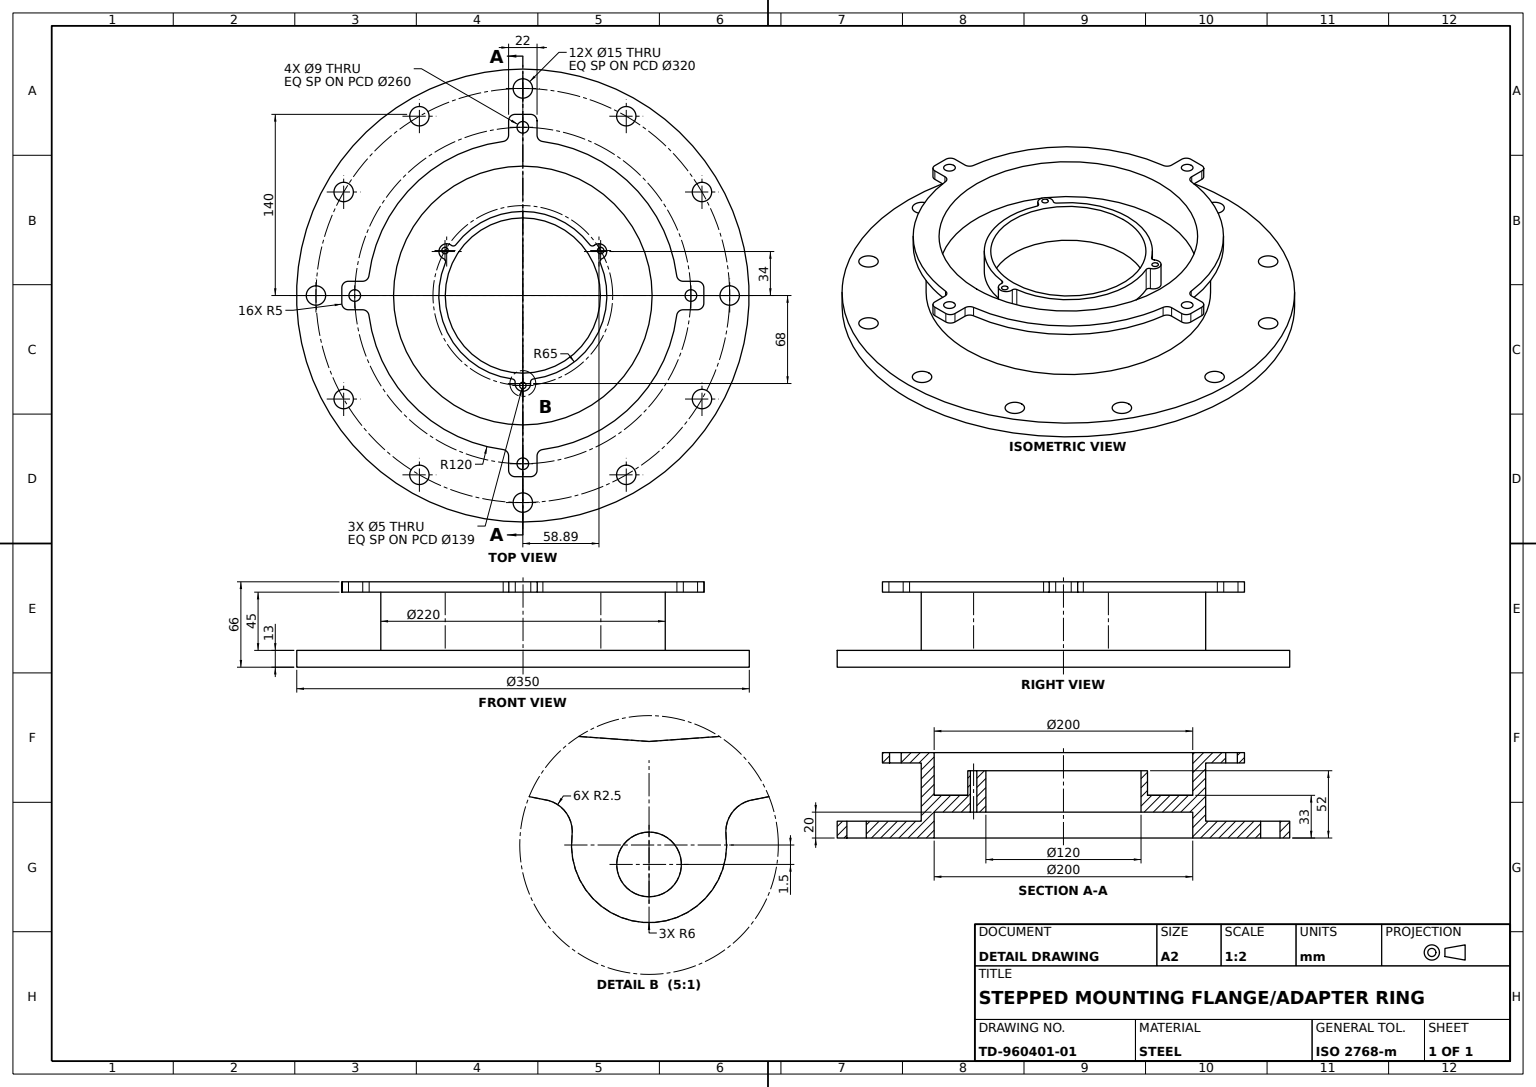
solid
v1 (60.188766,52,-37.25)
v2 (60.188766,52,-32.25)
e1 v1 v2 CIRCLE(AX(P(60.188766,52,-34.75),D(0,1,0),D(0,0,1)),2.5)
v3 (60.188766,20,-32.25)
e2 v3 v2 LINE
v4 (60.188766,20,-37.25)
e3 v3 v4 CIRCLE(AX(P(60.188766,20,-34.75),D(0,-1,0),D(0,0,-1)),2.5)
e4 v4 v1 LINE
face CYL(AX(P(60.188766,4,-34.75),D(0,1,0),D(0,0,1)),2.5) rev [e1 -e2 e3 e4]
v5 (0,58,110)
v6 (0,13,110)
e5 v5 v6 LINE
v7 (0,58,-110)
e6 v7 v5 CIRCLE(AX(P(0,58,0),D(0,1,0),D(0,0,1)),110)
v8 (0,13,-110)
e7 v7 v8 LINE
e8 v8 v6 CIRCLE(AX(P(0,13,0),D(0,1,0),D(0,0,1)),110)
face CYL(AX(P(0,58,0),D(0,-1,0),D(0,0,-1)),110) [-e5 -e6 e7 e8]
v9 (135,58,11.000001)
v10 (140,58,6.000001)
e9 v9 v10 CIRCLE(AX(P(135,58,6.000001),D(0,1,0),D(0,0,-1)),5)
v11 (140,66,6.000001)
e10 v11 v10 LINE
v12 (135,66,11.000001)
e11 v12 v11 CIRCLE(AX(P(135,66,6.000001),D(0,1,0),D(0,0,-1)),5)
e12 v12 v9 LINE
face CYL(AX(P(135,66,6.000001),D(0,-1,0),D(0,0,-1)),5) [e9 -e10 -e11 e12]
v13 (5.955837,33,67.273356)
v14 (-5.955837,33,67.273356)
e13 v13 v14 CIRCLE(AX(P(0,33,68),D(0,-1,0),D(0,0,-1)),6)
v15 (5.955837,52,67.273356)
e14 v15 v13 LINE
v16 (-5.955837,52,67.273356)
e15 v15 v16 CIRCLE(AX(P(0,52,68),D(0,-1,0),D(0,0,-1)),6)
e16 v16 v14 LINE
face CYL(AX(P(0,52,68),D(0,-1,0),D(0,0,-1)),6) [-e13 -e14 e15 e16]
v17 (130,58,4.5)
v18 (130,58,-4.5)
e17 v17 v18 CIRCLE(AX(P(130,58,0),D(0,-1,0),D(0,0,-1)),4.5)
e18 v18 v17 CIRCLE(AX(P(130,58,0),D(0,-1,0),D(0,0,-1)),4.5)
v19 (0,58,134.5)
v20 (0,58,125.5)
e19 v19 v20 CIRCLE(AX(P(0,58,130),D(0,-1,0),D(0,0,-1)),4.5)
e20 v20 v19 CIRCLE(AX(P(0,58,130),D(0,-1,0),D(0,0,-1)),4.5)
e21 v5 v7 CIRCLE(AX(P(0,58,0),D(0,1,0),D(0,0,1)),110)
v21 (0,58,-134.5)
v22 (0,58,-125.5)
e22 v21 v22 CIRCLE(AX(P(0,58,-130),D(0,-1,0),D(0,0,-1)),4.5)
e23 v22 v21 CIRCLE(AX(P(0,58,-130),D(0,-1,0),D(0,0,-1)),4.5)
v23 (-130,58,-4.5)
v24 (-130,58,4.5)
e24 v23 v24 CIRCLE(AX(P(-130,58,0),D(0,-1,0),D(0,0,-1)),4.5)
e25 v24 v23 CIRCLE(AX(P(-130,58,0),D(0,-1,0),D(0,0,-1)),4.5)
v25 (123.971771,58,11.000001)
e26 v25 v9 LINE
v26 (119.0129,58,15.360001)
e27 v26 v25 CIRCLE(AX(P(123.971771,58,16.000001),D(0,-1,0),D(0,0,1)),5)
v27 (15.36,58,119.0129)
e28 v27 v26 CIRCLE(AX(P(0,58,0),D(0,1,0),D(0,0,1)),120)
v28 (11,58,123.971771)
e29 v28 v27 CIRCLE(AX(P(16,58,123.971771),D(0,-1,0),D(0,0,-1)),5)
v29 (11,58,135)
e30 v29 v28 LINE
v30 (6,58,140)
e31 v30 v29 CIRCLE(AX(P(6,58,135),D(0,1,0),D(0,0,-1)),5)
v31 (-6.000001,58,140)
e32 v31 v30 LINE
v32 (-11.000001,58,135)
e33 v32 v31 CIRCLE(AX(P(-6.000001,58,135),D(0,1,0),D(0,0,-1)),5)
v33 (-11.000001,58,123.971771)
e34 v33 v32 LINE
v34 (-15.360001,58,119.0129)
e35 v34 v33 CIRCLE(AX(P(-16.000001,58,123.971771),D(0,-1,0),D(0,0,1)),5)
v35 (-119.0129,58,15.36)
e36 v35 v34 CIRCLE(AX(P(0,58,0),D(0,1,0),D(0,0,1)),120)
v36 (-123.971771,58,11)
e37 v36 v35 CIRCLE(AX(P(-123.971771,58,16),D(0,-1,0),D(0,0,-1)),5)
v37 (-135,58,11)
e38 v37 v36 LINE
v38 (-140,58,6)
e39 v38 v37 CIRCLE(AX(P(-135,58,6),D(0,1,0),D(0,0,-1)),5)
v39 (-140,58,-6.000001)
e40 v39 v38 LINE
v40 (-135,58,-11.000001)
e41 v40 v39 CIRCLE(AX(P(-135,58,-6.000001),D(0,1,0),D(0,0,-1)),5)
v41 (-123.971771,58,-11.000001)
e42 v41 v40 LINE
v42 (-119.0129,58,-15.360001)
e43 v42 v41 CIRCLE(AX(P(-123.971771,58,-16.000001),D(0,-1,0),D(0,0,1)),5)
v43 (-15.36,58,-119.0129)
e44 v43 v42 CIRCLE(AX(P(0,58,0),D(0,1,0),D(0,0,1)),120)
v44 (-11,58,-123.971771)
e45 v44 v43 CIRCLE(AX(P(-16,58,-123.971771),D(0,-1,0),D(0,0,-1)),5)
v45 (-11,58,-135)
e46 v45 v44 LINE
v46 (-6,58,-140)
e47 v46 v45 CIRCLE(AX(P(-6,58,-135),D(0,1,0),D(0,0,-1)),5)
v47 (6.000001,58,-140)
e48 v47 v46 LINE
v48 (11.000001,58,-135)
e49 v48 v47 CIRCLE(AX(P(6.000001,58,-135),D(0,1,0),D(0,0,-1)),5)
v49 (11.000001,58,-123.971771)
e50 v49 v48 LINE
v50 (15.360001,58,-119.0129)
e51 v50 v49 CIRCLE(AX(P(16.000001,58,-123.971771),D(0,-1,0),D(0,0,1)),5)
v51 (119.0129,58,-15.36)
e52 v51 v50 CIRCLE(AX(P(0,58,0),D(0,1,0),D(0,0,1)),120)
v52 (123.971771,58,-11)
e53 v52 v51 CIRCLE(AX(P(123.971771,58,-16),D(0,-1,0),D(0,0,-1)),5)
v53 (135,58,-11)
e54 v53 v52 LINE
v54 (140,58,-6)
e55 v54 v53 CIRCLE(AX(P(135,58,-6),D(0,1,0),D(0,0,-1)),5)
e56 v10 v54 LINE
face PLANE(AX(P(6.000001,58,-135),D(0,-1,0),D(0,0,-1))) [-e17 -e18] [-e19 -e20] [e21 e6] [-e22 -e23] [-e24 -e25] [-e26 -e27 -e28 -e29 -e30 -e31 -e32 -e33 -e34 -e35 -e36 -e37 -e38 -e39 -e40 -e41 -e42 -e43 -e44 -e45 -e46 -e47 -e48 -e49 -e50 -e51 -e52 -e53 -e54 -e55 -e56 -e9]
v55 (-160,0,7.5)
v56 (-160,13,7.5)
e57 v55 v56 LINE
v57 (-160,13,-7.5)
e58 v56 v57 CIRCLE(AX(P(-160,13,0),D(0,1,0),D(0,0,1)),7.5)
v58 (-160,0,-7.5)
e59 v58 v57 LINE
e60 v55 v58 CIRCLE(AX(P(-160,0,0),D(0,1,0),D(0,0,1)),7.5)
face CYL(AX(P(-160,-98,0),D(0,1,0),D(0,0,1)),7.5) rev [e57 e58 -e59 -e60]
v59 (-80,0,-146.064065)
v60 (-80,13,-146.064065)
e61 v59 v60 LINE
v61 (-80,13,-131.064065)
e62 v60 v61 CIRCLE(AX(P(-80,13,-138.564065),D(0,1,0),D(0,0,1)),7.5)
v62 (-80,0,-131.064065)
e63 v62 v61 LINE
e64 v59 v62 CIRCLE(AX(P(-80,0,-138.564065),D(0,1,0),D(0,0,1)),7.5)
face CYL(AX(P(-80,-98,-138.564065),D(0,1,0),D(0,0,1)),7.5) rev [e61 e62 -e63 -e64]
v63 (130,66,4.5)
e65 v17 v63 LINE
v64 (130,66,-4.5)
e66 v63 v64 CIRCLE(AX(P(130,66,0),D(0,1,0),D(0,0,1)),4.5)
e67 v18 v64 LINE
face CYL(AX(P(130,18,0),D(0,1,0),D(0,0,1)),4.5) rev [e65 e66 -e67 e18]
v65 (-15.36,66,-119.0129)
e68 v65 v43 LINE
v66 (-11,66,-123.971771)
e69 v66 v65 CIRCLE(AX(P(-16,66,-123.971771),D(0,-1,0),D(0,0,-1)),5)
e70 v66 v44 LINE
face CYL(AX(P(-16,66,-123.971771),D(0,-1,0),D(0,0,-1)),5) rev [e45 -e68 -e69 e70]
v67 (11.000001,66,-123.971771)
e71 v67 v49 LINE
v68 (11.000001,66,-135)
e72 v68 v48 LINE
e73 v67 v68 LINE
face PLANE(AX(P(11.000001,66,-135),D(-1,0,0),D(0,0,1))) rev [e71 e50 -e72 -e73]
v69 (80,13,-146.064065)
v70 (80,13,-131.064065)
e74 v69 v70 CIRCLE(AX(P(80,13,-138.564065),D(0,1,0),D(0,0,1)),7.5)
v71 (80,0,-131.064065)
e75 v71 v70 LINE
v72 (80,0,-146.064065)
e76 v72 v71 CIRCLE(AX(P(80,0,-138.564065),D(0,1,0),D(0,0,1)),7.5)
e77 v72 v69 LINE
face CYL(AX(P(80,-98,-138.564065),D(0,1,0),D(0,0,1)),7.5) rev [e74 -e75 -e76 e77]
v73 (-135,66,-11.000001)
e78 v73 v40 LINE
v74 (-123.971771,66,-11.000001)
e79 v74 v73 LINE
e80 v74 v41 LINE
face PLANE(AX(P(-135,66,-11.000001),D(0,0,1),D(1,0,0))) rev [e42 -e78 -e79 e80]
v75 (-130,66,4.5)
e81 v24 v75 LINE
v76 (-130,66,-4.5)
e82 v75 v76 CIRCLE(AX(P(-130,66,0),D(0,1,0),D(0,0,1)),4.5)
e83 v23 v76 LINE
face CYL(AX(P(-130,18,0),D(0,1,0),D(0,0,1)),4.5) rev [e24 e81 e82 -e83]
v77 (-55.282517,52,-38.794584)
v78 (-51.787679,52,-39.2815)
e84 v77 v78 CIRCLE(AX(P(-53.779513,52,-40.792327),D(0,1,0),D(0,0,1)),2.5)
v79 (-51.787679,33,-39.2815)
e85 v78 v79 LINE
v80 (-55.282517,33,-38.794584)
e86 v80 v79 CIRCLE(AX(P(-53.779513,33,-40.792327),D(0,1,0),D(0,0,-1)),2.5)
e87 v77 v80 LINE
face CYL(AX(P(-53.779513,52,-40.792327),D(0,-1,0),D(0,0,-1)),2.5) rev [e84 e85 -e86 -e87]
v81 (6.000001,66,-140)
e88 v81 v47 LINE
e89 v68 v81 CIRCLE(AX(P(6.000001,66,-135),D(0,1,0),D(0,0,-1)),5)
face CYL(AX(P(6.000001,66,-135),D(0,-1,0),D(0,0,-1)),5) [e72 e49 -e88 -e89]
v82 (138.564065,13,87.5)
v83 (138.564065,13,72.5)
e90 v82 v83 CIRCLE(AX(P(138.564065,13,80),D(0,1,0),D(0,0,1)),7.5)
v84 (138.564065,0,72.5)
e91 v84 v83 LINE
v85 (138.564065,0,87.5)
e92 v85 v84 CIRCLE(AX(P(138.564065,0,80),D(0,1,0),D(0,0,1)),7.5)
e93 v85 v82 LINE
face CYL(AX(P(138.564065,-98,80),D(0,1,0),D(0,0,1)),7.5) rev [e90 -e91 -e92 e93]
v86 (-58.889727,52,-40)
v87 (-58.889727,33,-40)
e94 v86 v87 LINE
e95 v86 v77 CIRCLE(AX(P(-58.889727,52,-34),D(0,-1,0),D(0,0,-1)),6)
e96 v87 v80 CIRCLE(AX(P(-58.889727,33,-34),D(0,-1,0),D(0,0,-1)),6)
face CYL(AX(P(-58.889727,52,-34),D(0,-1,0),D(0,0,-1)),6) [-e94 e95 e87 -e96]
v88 (0,66,125.5)
e97 v20 v88 LINE
v89 (0,66,134.5)
e98 v88 v89 CIRCLE(AX(P(0,66,130),D(0,1,0),D(0,0,1)),4.5)
e99 v19 v89 LINE
face CYL(AX(P(0,18,130),D(0,1,0),D(0,0,1)),4.5) rev [e97 e98 -e99 e19]
v90 (58.889727,33,-40)
v91 (61.238354,33,-28.478772)
e100 v90 v91 CIRCLE(AX(P(58.889727,33,-34),D(0,-1,0),D(0,0,-1)),6)
v92 (58.889727,52,-40)
e101 v92 v90 LINE
v93 (61.238354,52,-28.478772)
e102 v92 v93 CIRCLE(AX(P(58.889727,52,-34),D(0,-1,0),D(0,0,-1)),6)
e103 v93 v91 LINE
face CYL(AX(P(58.889727,52,-34),D(0,-1,0),D(0,0,-1)),6) [-e100 -e101 e102 e103]
v94 (0,20,-60)
v95 (0,52,-60)
e104 v94 v95 LINE
v96 (0,52,60)
e105 v95 v96 CIRCLE(AX(P(0,52,0),D(0,1,0),D(0,0,1)),60)
v97 (0,20,60)
e106 v97 v96 LINE
e107 v97 v94 CIRCLE(AX(P(0,20,0),D(0,-1,0),D(0,0,-1)),60)
face CYL(AX(P(0,-10,0),D(0,1,0),D(0,0,1)),60) rev [e104 e105 -e106 e107]
v98 (0,0,100)
v99 (0,0,-100)
e108 v98 v99 CIRCLE(AX(P(0,0,0),D(0,-1,0),D(0,0,-1)),100)
e109 v99 v98 CIRCLE(AX(P(0,0,0),D(0,-1,0),D(0,0,-1)),100)
v100 (-138.564065,0,-87.5)
v101 (-138.564065,0,-72.5)
e110 v100 v101 CIRCLE(AX(P(-138.564065,0,-80),D(0,1,0),D(0,0,1)),7.5)
e111 v101 v100 CIRCLE(AX(P(-138.564065,0,-80),D(0,1,0),D(0,0,1)),7.5)
v102 (0,0,-152.5)
v103 (0,0,-167.5)
e112 v102 v103 CIRCLE(AX(P(0,0,-160),D(0,1,0),D(0,0,1)),7.5)
e113 v103 v102 CIRCLE(AX(P(0,0,-160),D(0,1,0),D(0,0,1)),7.5)
v104 (138.564065,0,-87.5)
v105 (138.564065,0,-72.5)
e114 v104 v105 CIRCLE(AX(P(138.564065,0,-80),D(0,1,0),D(0,0,1)),7.5)
e115 v105 v104 CIRCLE(AX(P(138.564065,0,-80),D(0,1,0),D(0,0,1)),7.5)
v106 (80,0,131.064065)
v107 (80,0,146.064065)
e116 v106 v107 CIRCLE(AX(P(80,0,138.564065),D(0,1,0),D(0,0,1)),7.5)
e117 v107 v106 CIRCLE(AX(P(80,0,138.564065),D(0,1,0),D(0,0,1)),7.5)
e118 v58 v55 CIRCLE(AX(P(-160,0,0),D(0,1,0),D(0,0,1)),7.5)
e119 v71 v72 CIRCLE(AX(P(80,0,-138.564065),D(0,1,0),D(0,0,1)),7.5)
e120 v62 v59 CIRCLE(AX(P(-80,0,-138.564065),D(0,1,0),D(0,0,1)),7.5)
e121 v84 v85 CIRCLE(AX(P(138.564065,0,80),D(0,1,0),D(0,0,1)),7.5)
v108 (-80,0,146.064065)
v109 (-80,0,131.064065)
e122 v108 v109 CIRCLE(AX(P(-80,0,138.564065),D(0,1,0),D(0,0,1)),7.5)
e123 v109 v108 CIRCLE(AX(P(-80,0,138.564065),D(0,1,0),D(0,0,1)),7.5)
v110 (-138.564065,0,87.5)
v111 (-138.564065,0,72.5)
e124 v110 v111 CIRCLE(AX(P(-138.564065,0,80),D(0,1,0),D(0,0,1)),7.5)
e125 v111 v110 CIRCLE(AX(P(-138.564065,0,80),D(0,1,0),D(0,0,1)),7.5)
v112 (160,0,-7.5)
v113 (160,0,7.5)
e126 v112 v113 CIRCLE(AX(P(160,0,0),D(0,1,0),D(0,0,1)),7.5)
e127 v113 v112 CIRCLE(AX(P(160,0,0),D(0,1,0),D(0,0,1)),7.5)
v114 (0,0,175)
v115 (0,0,-175)
e128 v114 v115 CIRCLE(AX(P(0,0,0),D(0,1,0),D(0,0,1)),175)
e129 v115 v114 CIRCLE(AX(P(0,0,0),D(0,1,0),D(0,0,1)),175)
v116 (0,0,167.5)
v117 (0,0,152.5)
e130 v116 v117 CIRCLE(AX(P(0,0,160),D(0,1,0),D(0,0,1)),7.5)
e131 v117 v116 CIRCLE(AX(P(0,0,160),D(0,1,0),D(0,0,1)),7.5)
face PLANE(AX(P(0,0,0),D(0,1,0),D(0,0,1))) rev [-e108 -e109] [e110 e111] [e112 e113] [e114 e115] [e116 e117] [e60 e118] [e76 e119] [e64 e120] [e121 e92] [e122 e123] [e124 e125] [e126 e127] [-e128 -e129] [e130 e131]
v118 (6,66,140)
e132 v118 v30 LINE
v119 (-6.000001,66,140)
e133 v119 v118 LINE
e134 v119 v31 LINE
face PLANE(AX(P(6,66,140),D(0,0,-1),D(-1,0,0))) rev [-e132 -e133 e134 e32]
e135 v76 v75 CIRCLE(AX(P(-130,66,0),D(0,1,0),D(0,0,1)),4.5)
face CYL(AX(P(-130,18,0),D(0,1,0),D(0,0,1)),4.5) rev [-e81 e25 e83 e135]
v120 (0,66,-100)
v121 (0,33,-100)
e136 v120 v121 LINE
v122 (0,33,100)
e137 v121 v122 CIRCLE(AX(P(0,33,0),D(0,-1,0),D(0,0,-1)),100)
v123 (0,66,100)
e138 v123 v122 LINE
e139 v120 v123 CIRCLE(AX(P(0,66,0),D(0,-1,0),D(0,0,-1)),100)
face CYL(AX(P(0,86,0),D(0,-1,0),D(0,0,-1)),100) rev [e136 e137 -e138 -e139]
v124 (0,20,100)
e140 v124 v98 LINE
v125 (0,20,-100)
e141 v125 v124 CIRCLE(AX(P(0,20,0),D(0,-1,0),D(0,0,-1)),100)
e142 v125 v99 LINE
face CYL(AX(P(0,20,0),D(0,-1,0),D(0,0,-1)),100) rev [e109 -e140 -e141 e142]
v126 (-8.124938,52,64.490196)
e143 v16 v126 CIRCLE(AX(P(-8.437435,52,66.970588),D(0,1,0),D(0,0,1)),2.5)
v127 (-8.124938,33,64.490196)
e144 v126 v127 LINE
e145 v14 v127 CIRCLE(AX(P(-8.437435,33,66.970588),D(0,1,0),D(0,0,-1)),2.5)
face CYL(AX(P(-8.437435,52,66.970588),D(0,-1,0),D(0,0,-1)),2.5) rev [-e16 e143 e144 -e145]
v128 (-61.238354,52,-28.478772)
v129 (-61.238354,33,-28.478772)
e146 v128 v129 LINE
v130 (-59.912617,33,-25.208696)
e147 v130 v129 CIRCLE(AX(P(-62.216948,33,-26.178261),D(0,1,0),D(0,0,-1)),2.5)
v131 (-59.912617,52,-25.208696)
e148 v131 v130 LINE
e149 v131 v128 CIRCLE(AX(P(-62.216948,52,-26.178261),D(0,1,0),D(0,0,-1)),2.5)
face CYL(AX(P(-62.216948,52,-26.178261),D(0,-1,0),D(0,0,-1)),2.5) rev [e146 -e147 -e148 e149]
v132 (0,13,-175)
e150 v132 v115 LINE
v133 (0,13,175)
e151 v133 v132 CIRCLE(AX(P(0,13,0),D(0,1,0),D(0,0,1)),175)
e152 v133 v114 LINE
face CYL(AX(P(0,13,0),D(0,-1,0),D(0,0,-1)),175) [e128 -e150 -e151 e152]
v134 (0,66,-125.5)
v135 (0,66,-134.5)
e153 v134 v135 CIRCLE(AX(P(0,66,-130),D(0,1,0),D(0,0,1)),4.5)
e154 v21 v135 LINE
e155 v22 v134 LINE
face CYL(AX(P(0,18,-130),D(0,1,0),D(0,0,1)),4.5) rev [e153 -e154 e22 e155]
v136 (-135,66,11)
e156 v136 v37 LINE
v137 (-140,66,6)
e157 v137 v136 CIRCLE(AX(P(-135,66,6),D(0,1,0),D(0,0,-1)),5)
e158 v137 v38 LINE
face CYL(AX(P(-135,66,6),D(0,-1,0),D(0,0,-1)),5) [-e156 -e157 e158 e39]
v138 (160,13,-7.5)
e159 v112 v138 LINE
v139 (160,13,7.5)
e160 v113 v139 LINE
e161 v139 v138 CIRCLE(AX(P(160,13,0),D(0,1,0),D(0,0,1)),7.5)
face CYL(AX(P(160,-98,0),D(0,1,0),D(0,0,1)),7.5) rev [-e159 -e127 e160 e161]
v140 (-6,66,-140)
e162 v140 v46 LINE
e163 v81 v140 LINE
face PLANE(AX(P(-6,66,-140),D(0,0,1),D(1,0,0))) rev [e88 e48 -e162 -e163]
v141 (140,66,-6)
e164 v141 v54 LINE
v142 (135,66,-11)
e165 v142 v53 LINE
e166 v141 v142 CIRCLE(AX(P(135,66,-6),D(0,1,0),D(0,0,-1)),5)
face CYL(AX(P(135,66,-6),D(0,-1,0),D(0,0,-1)),5) [e164 e55 -e165 -e166]
v143 (-80,13,131.064065)
e167 v109 v143 LINE
v144 (-80,13,146.064065)
e168 v143 v144 CIRCLE(AX(P(-80,13,138.564065),D(0,1,0),D(0,0,1)),7.5)
e169 v108 v144 LINE
face CYL(AX(P(-80,-98,138.564065),D(0,1,0),D(0,0,1)),7.5) rev [-e123 e167 e168 -e169]
v145 (-60.188766,20,-32.25)
v146 (-60.188766,52,-32.25)
e170 v145 v146 LINE
v147 (-60.188766,20,-37.25)
e171 v145 v147 CIRCLE(AX(P(-60.188766,20,-34.75),D(0,-1,0),D(0,0,-1)),2.5)
v148 (-60.188766,52,-37.25)
e172 v147 v148 LINE
e173 v148 v146 CIRCLE(AX(P(-60.188766,52,-34.75),D(0,1,0),D(0,0,1)),2.5)
face CYL(AX(P(-60.188766,4,-34.75),D(0,1,0),D(0,0,1)),2.5) rev [-e170 e171 e172 e173]
v149 (15.36,66,119.0129)
e174 v149 v27 LINE
v150 (11,66,123.971771)
e175 v150 v149 CIRCLE(AX(P(16,66,123.971771),D(0,-1,0),D(0,0,-1)),5)
e176 v150 v28 LINE
face CYL(AX(P(16,66,123.971771),D(0,-1,0),D(0,0,-1)),5) rev [-e174 -e175 e176 e29]
e177 v89 v88 CIRCLE(AX(P(0,66,130),D(0,1,0),D(0,0,1)),4.5)
e178 v135 v134 CIRCLE(AX(P(0,66,-130),D(0,1,0),D(0,0,1)),4.5)
e179 v64 v63 CIRCLE(AX(P(130,66,0),D(0,1,0),D(0,0,1)),4.5)
e180 v123 v120 CIRCLE(AX(P(0,66,0),D(0,-1,0),D(0,0,-1)),100)
e181 v11 v141 LINE
v151 (123.971771,66,-11)
e182 v142 v151 LINE
v152 (119.0129,66,-15.36)
e183 v151 v152 CIRCLE(AX(P(123.971771,66,-16),D(0,-1,0),D(0,0,-1)),5)
v153 (15.360001,66,-119.0129)
e184 v152 v153 CIRCLE(AX(P(0,66,0),D(0,1,0),D(0,0,1)),120)
e185 v153 v67 CIRCLE(AX(P(16.000001,66,-123.971771),D(0,-1,0),D(0,0,1)),5)
v154 (-11,66,-135)
e186 v140 v154 CIRCLE(AX(P(-6,66,-135),D(0,1,0),D(0,0,-1)),5)
e187 v154 v66 LINE
v155 (-119.0129,66,-15.360001)
e188 v65 v155 CIRCLE(AX(P(0,66,0),D(0,1,0),D(0,0,1)),120)
e189 v155 v74 CIRCLE(AX(P(-123.971771,66,-16.000001),D(0,-1,0),D(0,0,1)),5)
v156 (-140,66,-6.000001)
e190 v73 v156 CIRCLE(AX(P(-135,66,-6.000001),D(0,1,0),D(0,0,-1)),5)
e191 v156 v137 LINE
v157 (-123.971771,66,11)
e192 v136 v157 LINE
v158 (-119.0129,66,15.36)
e193 v157 v158 CIRCLE(AX(P(-123.971771,66,16),D(0,-1,0),D(0,0,-1)),5)
v159 (-15.360001,66,119.0129)
e194 v158 v159 CIRCLE(AX(P(0,66,0),D(0,1,0),D(0,0,1)),120)
v160 (-11.000001,66,123.971771)
e195 v159 v160 CIRCLE(AX(P(-16.000001,66,123.971771),D(0,-1,0),D(0,0,1)),5)
v161 (-11.000001,66,135)
e196 v160 v161 LINE
e197 v161 v119 CIRCLE(AX(P(-6.000001,66,135),D(0,1,0),D(0,0,-1)),5)
v162 (11,66,135)
e198 v118 v162 CIRCLE(AX(P(6,66,135),D(0,1,0),D(0,0,-1)),5)
e199 v162 v150 LINE
v163 (119.0129,66,15.360001)
e200 v149 v163 CIRCLE(AX(P(0,66,0),D(0,1,0),D(0,0,1)),120)
v164 (123.971771,66,11.000001)
e201 v163 v164 CIRCLE(AX(P(123.971771,66,16.000001),D(0,-1,0),D(0,0,1)),5)
e202 v164 v12 LINE
face PLANE(AX(P(6.000001,66,-135),D(0,-1,0),D(0,0,-1))) rev [-e177 -e98] [-e153 -e178] [-e179 -e66] [e180 e139] [-e82 -e135] [e181 e166 e182 e183 e184 e185 e73 e89 e163 e186 e187 e69 e188 e189 e79 e190 e191 e157 e192 e193 e194 e195 e196 e197 e133 e198 e199 e175 e200 e201 e202 e11]
e203 v122 v121 CIRCLE(AX(P(0,33,0),D(0,-1,0),D(0,0,-1)),100)
face CYL(AX(P(0,86,0),D(0,-1,0),D(0,0,-1)),100) rev [-e180 e138 e203 -e136]
e204 v2 v1 CIRCLE(AX(P(60.188766,52,-34.75),D(0,1,0),D(0,0,1)),2.5)
e205 v96 v95 CIRCLE(AX(P(0,52,0),D(0,1,0),D(0,0,1)),60)
v165 (0,52,72)
v166 (0,52,67)
e206 v165 v166 CIRCLE(AX(P(0,52,69.5),D(0,1,0),D(0,0,1)),2.5)
e207 v166 v165 CIRCLE(AX(P(0,52,69.5),D(0,1,0),D(0,0,1)),2.5)
e208 v146 v148 CIRCLE(AX(P(-60.188766,52,-34.75),D(0,1,0),D(0,0,1)),2.5)
v167 (51.787679,52,-39.2815)
v168 (55.282517,52,-38.794584)
e209 v167 v168 CIRCLE(AX(P(53.779513,52,-40.792327),D(0,1,0),D(0,0,-1)),2.5)
v169 (0,52,-65)
e210 v169 v167 CIRCLE(AX(P(0,52,0),D(0,-1,0),D(0,0,-1)),65)
e211 v78 v169 CIRCLE(AX(P(0,52,0),D(0,-1,0),D(0,0,-1)),65)
e212 v128 v86 CIRCLE(AX(P(-58.889727,52,-34),D(0,-1,0),D(0,0,-1)),6)
e213 v126 v131 CIRCLE(AX(P(0,52,0),D(0,-1,0),D(0,0,-1)),65)
v170 (8.124938,52,64.490196)
e214 v170 v15 CIRCLE(AX(P(8.437435,52,66.970588),D(0,1,0),D(0,0,-1)),2.5)
v171 (59.912617,52,-25.208696)
e215 v171 v170 CIRCLE(AX(P(0,52,0),D(0,-1,0),D(0,0,-1)),65)
e216 v93 v171 CIRCLE(AX(P(62.216948,52,-26.178261),D(0,1,0),D(0,0,1)),2.5)
e217 v168 v92 CIRCLE(AX(P(58.889727,52,-34),D(0,-1,0),D(0,0,-1)),6)
face PLANE(AX(P(-4.218718,52,33.485294),D(0,1,0),D(0,0,1))) [-e1 -e204] [-e105 -e205] [-e206 -e207] [-e173 -e208] [-e209 -e210 -e211 -e84 -e95 -e212 -e149 -e213 -e143 -e15 -e214 -e215 -e216 -e102 -e217]
v172 (0,33,-65)
v173 (51.787679,33,-39.2815)
e218 v172 v173 CIRCLE(AX(P(0,33,0),D(0,-1,0),D(0,0,-1)),65)
e219 v169 v172 LINE
e220 v167 v173 LINE
face CYL(AX(P(0,52,0),D(0,-1,0),D(0,0,-1)),65) [-e218 -e219 e210 e220]
v174 (8.124938,33,64.490196)
e221 v170 v174 LINE
v175 (59.912617,33,-25.208696)
e222 v175 v174 CIRCLE(AX(P(0,33,0),D(0,-1,0),D(0,0,-1)),65)
e223 v171 v175 LINE
face CYL(AX(P(0,52,0),D(0,-1,0),D(0,0,-1)),65) [e221 -e222 -e223 e215]
e224 v157 v36 LINE
face PLANE(AX(P(-123.971771,66,11),D(0,0,-1),D(-1,0,0))) rev [-e192 e156 e38 -e224]
v176 (-138.564065,13,87.5)
e225 v110 v176 LINE
v177 (-138.564065,13,72.5)
e226 v176 v177 CIRCLE(AX(P(-138.564065,13,80),D(0,1,0),D(0,0,1)),7.5)
e227 v111 v177 LINE
face CYL(AX(P(-138.564065,-98,80),D(0,1,0),D(0,0,1)),7.5) rev [-e124 e225 e226 -e227]
face CYL(AX(P(0,18,-130),D(0,1,0),D(0,0,1)),4.5) rev [-e155 e23 e154 e178]
e228 v4 v3 CIRCLE(AX(P(60.188766,20,-34.75),D(0,-1,0),D(0,0,-1)),2.5)
v178 (0,20,67)
v179 (0,20,72)
e229 v178 v179 CIRCLE(AX(P(0,20,69.5),D(0,-1,0),D(0,0,-1)),2.5)
e230 v179 v178 CIRCLE(AX(P(0,20,69.5),D(0,-1,0),D(0,0,-1)),2.5)
e231 v124 v125 CIRCLE(AX(P(0,20,0),D(0,-1,0),D(0,0,-1)),100)
e232 v94 v97 CIRCLE(AX(P(0,20,0),D(0,-1,0),D(0,0,-1)),60)
e233 v147 v145 CIRCLE(AX(P(-60.188766,20,-34.75),D(0,-1,0),D(0,0,-1)),2.5)
face PLANE(AX(P(0,20,0),D(0,-1,0),D(0,0,-1))) [-e228 -e3] [-e229 -e230] [e141 e231] [-e232 -e107] [-e233 -e171]
v180 (0,13,-152.5)
e234 v102 v180 LINE
v181 (0,13,-167.5)
e235 v103 v181 LINE
e236 v181 v180 CIRCLE(AX(P(0,13,-160),D(0,1,0),D(0,0,1)),7.5)
face CYL(AX(P(0,-98,-160),D(0,1,0),D(0,0,1)),7.5) rev [-e234 -e113 e235 e236]
face CYL(AX(P(130,18,0),D(0,1,0),D(0,0,1)),4.5) rev [-e65 e17 e67 e179]
v182 (0,13,152.5)
e237 v117 v182 LINE
v183 (0,13,167.5)
e238 v116 v183 LINE
e239 v183 v182 CIRCLE(AX(P(0,13,160),D(0,1,0),D(0,0,1)),7.5)
face CYL(AX(P(0,-98,160),D(0,1,0),D(0,0,1)),7.5) rev [-e237 -e130 e238 e239]
e240 v160 v33 LINE
e241 v159 v34 LINE
face CYL(AX(P(-16.000001,66,123.971771),D(0,-1,0),D(0,0,-1)),5) rev [-e240 -e195 e241 e35]
v184 (55.282517,33,-38.794584)
e242 v184 v90 CIRCLE(AX(P(58.889727,33,-34),D(0,-1,0),D(0,0,-1)),6)
e243 v168 v184 LINE
face CYL(AX(P(58.889727,52,-34),D(0,-1,0),D(0,0,-1)),6) [e101 -e242 -e243 e217]
face CYL(AX(P(0,20,0),D(0,-1,0),D(0,0,-1)),100) rev [e140 e108 -e142 -e231]
v185 (-138.564065,13,-72.5)
e244 v101 v185 LINE
v186 (-138.564065,13,-87.5)
e245 v185 v186 CIRCLE(AX(P(-138.564065,13,-80),D(0,1,0),D(0,0,1)),7.5)
e246 v100 v186 LINE
face CYL(AX(P(-138.564065,-98,-80),D(0,1,0),D(0,0,1)),7.5) rev [-e111 e244 e245 -e246]
e247 v154 v45 LINE
face PLANE(AX(P(-11,66,-123.971771),D(1,0,0),D(0,0,-1))) rev [-e70 -e187 e247 e46]
e248 v182 v183 CIRCLE(AX(P(0,13,160),D(0,1,0),D(0,0,1)),7.5)
face CYL(AX(P(0,-98,160),D(0,1,0),D(0,0,1)),7.5) rev [-e131 e237 e248 -e238]
face CYL(AX(P(60.188766,4,-34.75),D(0,1,0),D(0,0,1)),2.5) rev [-e4 e228 e2 e204]
e249 v162 v29 LINE
face PLANE(AX(P(11,66,123.971771),D(-1,0,0),D(0,0,1))) rev [e249 e30 -e176 -e199]
e250 v156 v39 LINE
face PLANE(AX(P(-140,66,6),D(1,0,0),D(0,0,-1))) rev [e250 e40 -e158 -e191]
e251 v163 v26 LINE
face CYL(AX(P(0,66,0),D(0,-1,0),D(0,0,-1)),120) [-e251 -e200 e174 e28]
e252 v164 v25 LINE
face PLANE(AX(P(135,66,11.000001),D(0,0,-1),D(-1,0,0))) rev [e26 -e12 -e202 e252]
e253 v174 v13 CIRCLE(AX(P(8.437435,33,66.970588),D(0,1,0),D(0,0,-1)),2.5)
face CYL(AX(P(8.437435,52,66.970588),D(0,-1,0),D(0,0,-1)),2.5) rev [-e253 -e221 e214 e14]
e254 v151 v52 LINE
e255 v152 v51 LINE
face CYL(AX(P(123.971771,66,-16),D(0,-1,0),D(0,0,-1)),5) rev [-e183 e254 e53 -e255]
e256 v186 v185 CIRCLE(AX(P(-138.564065,13,-80),D(0,1,0),D(0,0,1)),7.5)
v187 (80,13,146.064065)
v188 (80,13,131.064065)
e257 v187 v188 CIRCLE(AX(P(80,13,138.564065),D(0,1,0),D(0,0,1)),7.5)
e258 v188 v187 CIRCLE(AX(P(80,13,138.564065),D(0,1,0),D(0,0,1)),7.5)
e259 v177 v176 CIRCLE(AX(P(-138.564065,13,80),D(0,1,0),D(0,0,1)),7.5)
e260 v138 v139 CIRCLE(AX(P(160,13,0),D(0,1,0),D(0,0,1)),7.5)
e261 v61 v60 CIRCLE(AX(P(-80,13,-138.564065),D(0,1,0),D(0,0,1)),7.5)
e262 v144 v143 CIRCLE(AX(P(-80,13,138.564065),D(0,1,0),D(0,0,1)),7.5)
e263 v57 v56 CIRCLE(AX(P(-160,13,0),D(0,1,0),D(0,0,1)),7.5)
e264 v83 v82 CIRCLE(AX(P(138.564065,13,80),D(0,1,0),D(0,0,1)),7.5)
e265 v180 v181 CIRCLE(AX(P(0,13,-160),D(0,1,0),D(0,0,1)),7.5)
e266 v70 v69 CIRCLE(AX(P(80,13,-138.564065),D(0,1,0),D(0,0,1)),7.5)
e267 v6 v8 CIRCLE(AX(P(0,13,0),D(0,1,0),D(0,0,1)),110)
v189 (138.564065,13,-87.5)
v190 (138.564065,13,-72.5)
e268 v189 v190 CIRCLE(AX(P(138.564065,13,-80),D(0,1,0),D(0,0,1)),7.5)
e269 v190 v189 CIRCLE(AX(P(138.564065,13,-80),D(0,1,0),D(0,0,1)),7.5)
e270 v132 v133 CIRCLE(AX(P(0,13,0),D(0,1,0),D(0,0,1)),175)
face PLANE(AX(P(0,13,0),D(0,1,0),D(0,0,1))) [-e256 -e245] [-e257 -e258] [-e259 -e226] [-e260 -e161] [-e261 -e62] [-e168 -e262] [-e58 -e263] [-e248 -e239] [-e264 -e90] [-e265 -e236] [-e266 -e74] [-e267 -e8] [-e268 -e269] [e151 e270]
e271 v155 v42 LINE
face CYL(AX(P(-123.971771,66,-16.000001),D(0,-1,0),D(0,0,-1)),5) rev [e43 -e80 -e189 e271]
face CYL(AX(P(-160,-98,0),D(0,1,0),D(0,0,1)),7.5) rev [e263 -e57 -e118 e59]
face CYL(AX(P(138.564065,-98,80),D(0,1,0),D(0,0,1)),7.5) rev [-e93 -e121 e91 e264]
e272 v129 v87 CIRCLE(AX(P(-58.889727,33,-34),D(0,-1,0),D(0,0,-1)),6)
face CYL(AX(P(-58.889727,52,-34),D(0,-1,0),D(0,0,-1)),6) [e94 -e272 -e146 e212]
e273 v79 v172 CIRCLE(AX(P(0,33,0),D(0,-1,0),D(0,0,-1)),65)
e274 v173 v184 CIRCLE(AX(P(53.779513,33,-40.792327),D(0,1,0),D(0,0,-1)),2.5)
e275 v91 v175 CIRCLE(AX(P(62.216948,33,-26.178261),D(0,1,0),D(0,0,-1)),2.5)
e276 v127 v130 CIRCLE(AX(P(0,33,0),D(0,-1,0),D(0,0,-1)),65)
face PLANE(AX(P(0,33,0),D(0,-1,0),D(0,0,-1))) rev [-e137 -e203] [e86 e273 e218 e274 e242 e100 e275 e222 e253 e13 e145 e276 e147 e272 e96]
face CYL(AX(P(-6,66,-135),D(0,-1,0),D(0,0,-1)),5) [e47 -e247 -e186 e162]
face CYL(AX(P(6,66,135),D(0,-1,0),D(0,0,-1)),5) [-e249 -e198 e132 e31]
e277 v161 v32 LINE
face PLANE(AX(P(-11.000001,66,135),D(1,0,0),D(0,0,-1))) rev [-e277 -e196 e240 e34]
face CYL(AX(P(-80,-98,138.564065),D(0,1,0),D(0,0,1)),7.5) rev [e262 -e167 -e122 e169]
e278 v104 v189 LINE
e279 v105 v190 LINE
face CYL(AX(P(138.564065,-98,-80),D(0,1,0),D(0,0,1)),7.5) rev [-e278 -e115 e279 e269]
e280 v153 v50 LINE
face CYL(AX(P(16.000001,66,-123.971771),D(0,-1,0),D(0,0,-1)),5) rev [e51 -e71 -e185 e280]
face PLANE(AX(P(123.971771,66,-11),D(0,0,1),D(1,0,0))) rev [e54 -e254 -e182 e165]
e281 v179 v165 LINE
e282 v178 v166 LINE
face CYL(AX(P(0,4,69.5),D(0,1,0),D(0,0,1)),2.5) rev [e229 e281 e206 -e282]
face CYL(AX(P(138.564065,-98,-80),D(0,1,0),D(0,0,1)),7.5) rev [-e114 e278 e268 -e279]
face CYL(AX(P(0,58,0),D(0,-1,0),D(0,0,-1)),110) [-e7 -e21 e5 e267]
face CYL(AX(P(0,52,0),D(0,-1,0),D(0,0,-1)),65) [-e85 e211 e219 -e273]
e283 v106 v188 LINE
e284 v107 v187 LINE
face CYL(AX(P(80,-98,138.564065),D(0,1,0),D(0,0,1)),7.5) rev [-e283 -e117 e284 e257]
face CYL(AX(P(0,66,0),D(0,-1,0),D(0,0,-1)),120) [-e280 -e184 e255 e52]
face CYL(AX(P(0,13,0),D(0,-1,0),D(0,0,-1)),175) [e150 e129 -e152 -e270]
face CYL(AX(P(62.216948,52,-26.178261),D(0,-1,0),D(0,0,-1)),2.5) rev [e216 e223 -e275 -e103]
face CYL(AX(P(80,-98,-138.564065),D(0,1,0),D(0,0,1)),7.5) rev [-e119 e75 e266 -e77]
face CYL(AX(P(-138.564065,-98,-80),D(0,1,0),D(0,0,1)),7.5) rev [-e110 e246 e256 -e244]
face CYL(AX(P(160,-98,0),D(0,1,0),D(0,0,1)),7.5) rev [-e126 e159 e260 -e160]
face CYL(AX(P(-60.188766,4,-34.75),D(0,1,0),D(0,0,1)),2.5) rev [e233 e170 e208 -e172]
face CYL(AX(P(-135,66,-6.000001),D(0,-1,0),D(0,0,-1)),5) [e78 e41 -e250 -e190]
face CYL(AX(P(-80,-98,-138.564065),D(0,1,0),D(0,0,1)),7.5) rev [e261 -e61 -e120 e63]
face CYL(AX(P(80,-98,138.564065),D(0,1,0),D(0,0,1)),7.5) rev [e283 e258 -e284 -e116]
face PLANE(AX(P(140,66,-6),D(-1,0,0),D(0,0,1))) rev [e56 -e164 -e181 e10]
e285 v158 v35 LINE
face CYL(AX(P(-123.971771,66,16),D(0,-1,0),D(0,0,-1)),5) rev [-e285 -e193 e224 e37]
face CYL(AX(P(-138.564065,-98,80),D(0,1,0),D(0,0,1)),7.5) rev [e227 e259 -e225 -e125]
face CYL(AX(P(0,-98,-160),D(0,1,0),D(0,0,1)),7.5) rev [-e112 e234 e265 -e235]
face CYL(AX(P(0,4,69.5),D(0,1,0),D(0,0,1)),2.5) rev [e230 e282 e207 -e281]
face CYL(AX(P(53.779513,52,-40.792327),D(0,-1,0),D(0,0,-1)),2.5) rev [-e274 -e220 e209 e243]
face CYL(AX(P(0,66,0),D(0,-1,0),D(0,0,-1)),120) [-e188 e68 e44 -e271]
face CYL(AX(P(0,66,0),D(0,-1,0),D(0,0,-1)),120) [e285 e36 -e241 -e194]
face CYL(AX(P(123.971771,66,16.000001),D(0,-1,0),D(0,0,-1)),5) rev [e27 -e252 -e201 e251]
face CYL(AX(P(0,-10,0),D(0,1,0),D(0,0,1)),60) rev [-e104 e232 e106 e205]
face CYL(AX(P(0,52,0),D(0,-1,0),D(0,0,-1)),65) [-e144 e213 e148 -e276]
face CYL(AX(P(-6.000001,66,135),D(0,-1,0),D(0,0,-1)),5) [-e197 e277 e33 -e134]
face CYL(AX(P(0,18,130),D(0,1,0),D(0,0,1)),4.5) rev [e177 -e97 e20 e99]
